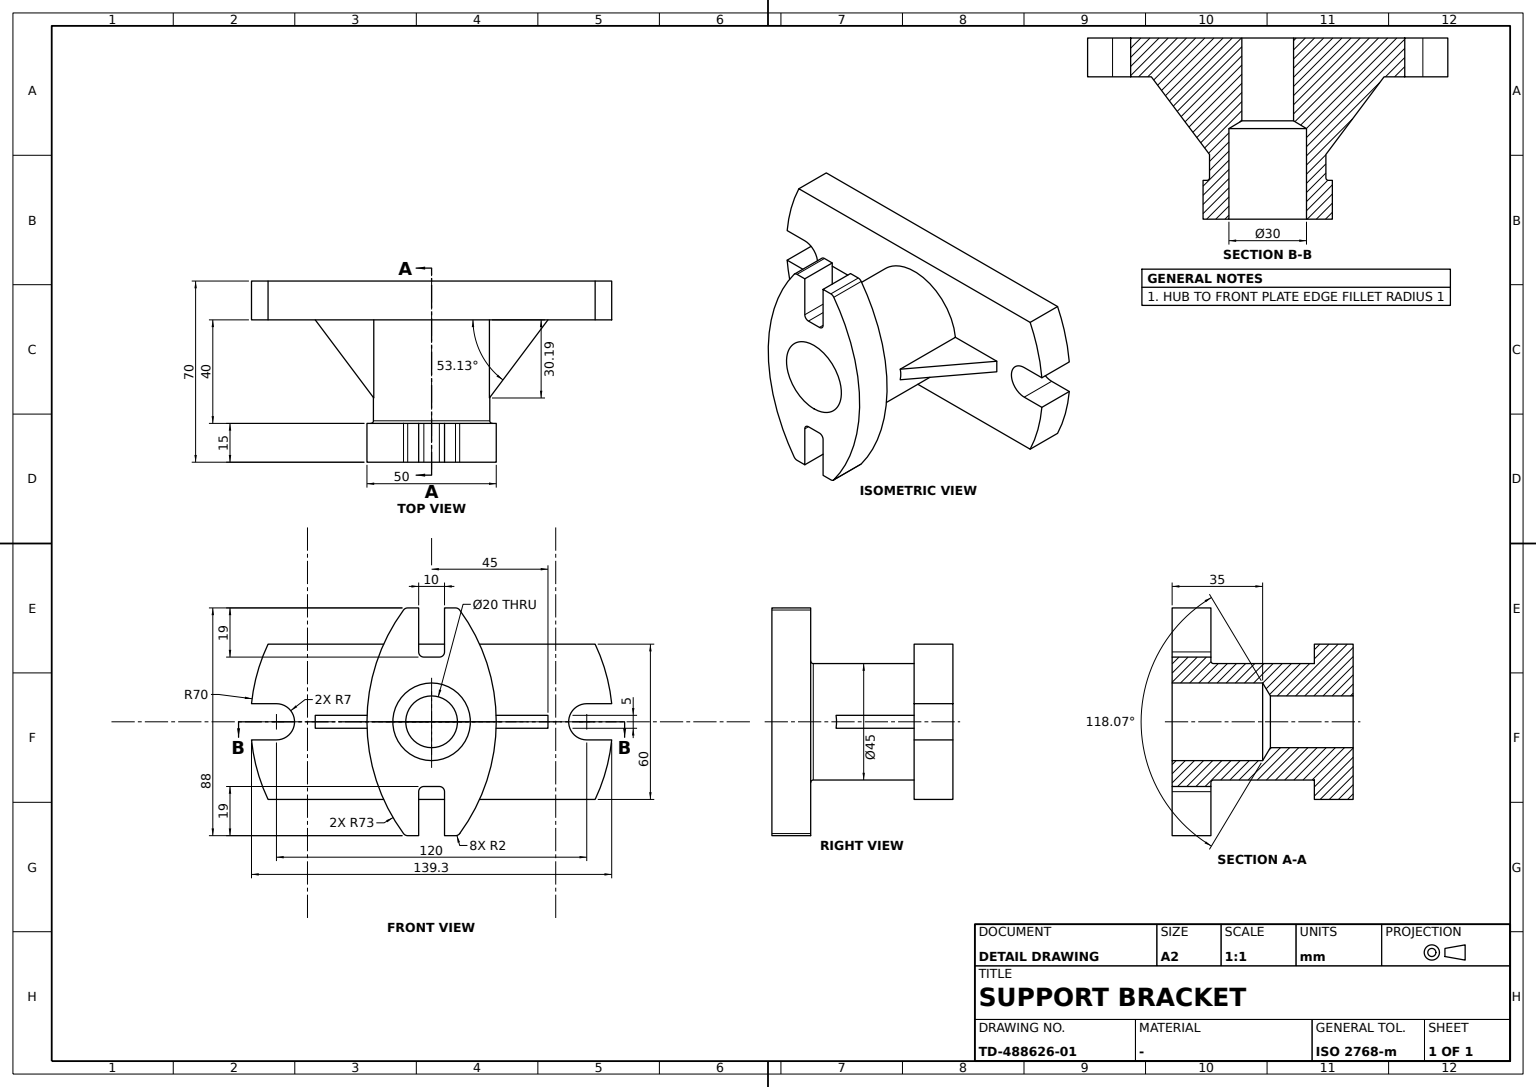
ISO-10303-21;
HEADER;
FILE_DESCRIPTION((''),'2;1');
FILE_NAME('','',(''),(''),'','','');
FILE_SCHEMA(('AUTOMOTIVE_DESIGN'));
ENDSEC;
DATA;
#1=APPLICATION_CONTEXT('');
#2=PRODUCT_CONTEXT('',#1,'mechanical');
#3=PRODUCT('','','',(#2));
#4=PRODUCT_DEFINITION_FORMATION('','',#3);
#5=PRODUCT_DEFINITION_CONTEXT('',#1,'design');
#6=PRODUCT_DEFINITION('','',#4,#5);
#7=PRODUCT_DEFINITION_SHAPE('','',#6);
#8=(LENGTH_UNIT()NAMED_UNIT(*)SI_UNIT(.MILLI.,.METRE.));
#9=(NAMED_UNIT(*)PLANE_ANGLE_UNIT()SI_UNIT($,.RADIAN.));
#10=(NAMED_UNIT(*)SI_UNIT($,.STERADIAN.)SOLID_ANGLE_UNIT());
#11=UNCERTAINTY_MEASURE_WITH_UNIT(LENGTH_MEASURE(0.005),#8,'distance_accuracy_value','');
#12=(GEOMETRIC_REPRESENTATION_CONTEXT(3)GLOBAL_UNCERTAINTY_ASSIGNED_CONTEXT((#11))GLOBAL_UNIT_ASSIGNED_CONTEXT((#8,#9,#10))REPRESENTATION_CONTEXT('',''));
#13=CARTESIAN_POINT('',(-7.5,-63.245553,30.));
#14=VERTEX_POINT('',#13);
#15=CARTESIAN_POINT('',(7.5,-63.245553,30.));
#16=VERTEX_POINT('',#15);
#17=DIRECTION('',(1.,0.,0.));
#18=VECTOR('',#17,1000.);
#19=LINE('',#13,#18);
#20=EDGE_CURVE('',#14,#16,#19,.T.);
#21=ORIENTED_EDGE('',*,*,#20,.F.);
#22=CARTESIAN_POINT('',(-7.5,-69.649121,7.));
#23=VERTEX_POINT('',#22);
#24=CARTESIAN_POINT('',(-7.5,0.,0.));
#25=DIRECTION('',(0.,0.,-1.));
#26=AXIS2_PLACEMENT_3D('',#24,#17,#25);
#27=CIRCLE('',#26,70.);
#28=EDGE_CURVE('',#14,#23,#27,.T.);
#29=ORIENTED_EDGE('',*,*,#28,.T.);
#30=CARTESIAN_POINT('',(7.5,-69.649121,7.));
#31=VERTEX_POINT('',#30);
#32=LINE('',#22,#18);
#33=EDGE_CURVE('',#23,#31,#32,.T.);
#34=ORIENTED_EDGE('',*,*,#33,.T.);
#35=CARTESIAN_POINT('',(7.5,0.,0.));
#36=AXIS2_PLACEMENT_3D('',#35,#17,#25);
#37=CIRCLE('',#36,70.);
#38=EDGE_CURVE('',#16,#31,#37,.T.);
#39=ORIENTED_EDGE('',*,*,#38,.F.);
#40=EDGE_LOOP('',(#21,#29,#34,#39));
#41=FACE_BOUND('',#40,.T.);
#42=CARTESIAN_POINT('',(0.,0.,0.));
#43=DIRECTION('',(0.,1.,0.));
#44=AXIS2_PLACEMENT_3D('',#42,#17,#43);
#45=CYLINDRICAL_SURFACE('',#44,70.);
#46=ADVANCED_FACE('',(#41),#45,.T.);
#47=CARTESIAN_POINT('',(7.5,63.245553,-30.));
#48=VERTEX_POINT('',#47);
#49=CARTESIAN_POINT('',(7.5,69.649121,-7.));
#50=VERTEX_POINT('',#49);
#51=EDGE_CURVE('',#48,#50,#37,.T.);
#52=ORIENTED_EDGE('',*,*,#51,.F.);
#53=CARTESIAN_POINT('',(-7.5,63.245553,-30.));
#54=VERTEX_POINT('',#53);
#55=LINE('',#53,#18);
#56=EDGE_CURVE('',#54,#48,#55,.T.);
#57=ORIENTED_EDGE('',*,*,#56,.F.);
#58=CARTESIAN_POINT('',(-7.5,69.649121,-7.));
#59=VERTEX_POINT('',#58);
#60=EDGE_CURVE('',#54,#59,#27,.T.);
#61=ORIENTED_EDGE('',*,*,#60,.T.);
#62=LINE('',#58,#18);
#63=EDGE_CURVE('',#59,#50,#62,.T.);
#64=ORIENTED_EDGE('',*,*,#63,.T.);
#65=EDGE_LOOP('',(#52,#57,#61,#64));
#66=FACE_BOUND('',#65,.T.);
#67=ADVANCED_FACE('',(#66),#45,.T.);
#68=CARTESIAN_POINT('',(62.5,-5.,-44.));
#69=VERTEX_POINT('',#68);
#70=CARTESIAN_POINT('',(47.5,-5.,-44.));
#71=VERTEX_POINT('',#70);
#72=DIRECTION('',(-1.,0.,0.));
#73=VECTOR('',#72,1000.);
#74=LINE('',#68,#73);
#75=EDGE_CURVE('',#69,#71,#74,.T.);
#76=ORIENTED_EDGE('',*,*,#75,.F.);
#77=CARTESIAN_POINT('',(62.5,-9.245087,-44.));
#78=VERTEX_POINT('',#77);
#79=CARTESIAN_POINT('',(62.5,0.,-44.));
#80=DIRECTION('',(0.,-1.,0.));
#81=VECTOR('',#80,1000.);
#82=LINE('',#79,#81);
#83=EDGE_CURVE('',#69,#78,#82,.T.);
#84=ORIENTED_EDGE('',*,*,#83,.T.);
#85=CARTESIAN_POINT('',(47.5,-9.245087,-44.));
#86=VERTEX_POINT('',#85);
#87=CARTESIAN_POINT('',(55.,-9.245087,-44.));
#88=LINE('',#87,#73);
#89=EDGE_CURVE('',#78,#86,#88,.T.);
#90=ORIENTED_EDGE('',*,*,#89,.T.);
#91=CARTESIAN_POINT('',(47.5,0.,-44.));
#92=LINE('',#91,#81);
#93=EDGE_CURVE('',#71,#86,#92,.T.);
#94=ORIENTED_EDGE('',*,*,#93,.F.);
#95=EDGE_LOOP('',(#76,#84,#90,#94));
#96=FACE_BOUND('',#95,.T.);
#97=CARTESIAN_POINT('',(62.5,5.,-44.));
#98=DIRECTION('',(0.,0.,1.));
#99=AXIS2_PLACEMENT_3D('',#97,#98,#43);
#100=PLANE('',#99);
#101=ADVANCED_FACE('',(#96),#100,.F.);
#102=VERTEX_POINT('',#97);
#103=CARTESIAN_POINT('',(47.5,5.,-44.));
#104=VERTEX_POINT('',#103);
#105=LINE('',#97,#73);
#106=EDGE_CURVE('',#102,#104,#105,.T.);
#107=ORIENTED_EDGE('',*,*,#106,.F.);
#108=CARTESIAN_POINT('',(62.5,5.,-27.));
#109=VERTEX_POINT('',#108);
#110=CARTESIAN_POINT('',(62.5,5.,-25.));
#111=VECTOR('',#25,1000.);
#112=LINE('',#110,#111);
#113=EDGE_CURVE('',#109,#102,#112,.T.);
#114=ORIENTED_EDGE('',*,*,#113,.F.);
#115=CARTESIAN_POINT('',(47.5,5.,-27.));
#116=VERTEX_POINT('',#115);
#117=CARTESIAN_POINT('',(55.,5.,-27.));
#118=LINE('',#117,#73);
#119=EDGE_CURVE('',#109,#116,#118,.T.);
#120=ORIENTED_EDGE('',*,*,#119,.T.);
#121=CARTESIAN_POINT('',(47.5,5.,-25.));
#122=LINE('',#121,#111);
#123=EDGE_CURVE('',#116,#104,#122,.T.);
#124=ORIENTED_EDGE('',*,*,#123,.T.);
#125=EDGE_LOOP('',(#107,#114,#120,#124));
#126=FACE_BOUND('',#125,.T.);
#127=AXIS2_PLACEMENT_3D('',#110,#43,#25);
#128=PLANE('',#127);
#129=ADVANCED_FACE('',(#126),#128,.F.);
#130=CARTESIAN_POINT('',(-7.5,0.,-10.));
#131=VERTEX_POINT('',#130);
#132=CIRCLE('',#26,10.);
#133=EDGE_CURVE('',#131,#131,#132,.T.);
#134=ORIENTED_EDGE('',*,*,#133,.F.);
#135=EDGE_LOOP('',(#134));
#136=FACE_BOUND('',#135,.T.);
#137=CARTESIAN_POINT('',(24.5,0.,-10.));
#138=VERTEX_POINT('',#137);
#139=CARTESIAN_POINT('',(24.5,0.,0.));
#140=AXIS2_PLACEMENT_3D('',#139,#17,#25);
#141=CIRCLE('',#140,10.);
#142=EDGE_CURVE('',#138,#138,#141,.T.);
#143=ORIENTED_EDGE('',*,*,#142,.T.);
#144=EDGE_LOOP('',(#143));
#145=FACE_BOUND('',#144,.T.);
#146=CARTESIAN_POINT('',(27.5,0.,0.));
#147=AXIS2_PLACEMENT_3D('',#146,#17,#43);
#148=CYLINDRICAL_SURFACE('',#147,10.);
#149=ADVANCED_FACE('',(#136,#145),#148,.F.);
#150=CARTESIAN_POINT('',(62.5,-3.,25.));
#151=VERTEX_POINT('',#150);
#152=CARTESIAN_POINT('',(62.5,3.,25.));
#153=VERTEX_POINT('',#152);
#154=CARTESIAN_POINT('',(62.5,-5.,25.));
#155=VECTOR('',#43,1000.);
#156=LINE('',#154,#155);
#157=EDGE_CURVE('',#151,#153,#156,.T.);
#158=ORIENTED_EDGE('',*,*,#157,.T.);
#159=CARTESIAN_POINT('',(47.5,3.,25.));
#160=VERTEX_POINT('',#159);
#161=CARTESIAN_POINT('',(55.,3.,25.));
#162=LINE('',#161,#73);
#163=EDGE_CURVE('',#153,#160,#162,.T.);
#164=ORIENTED_EDGE('',*,*,#163,.T.);
#165=CARTESIAN_POINT('',(47.5,-3.,25.));
#166=VERTEX_POINT('',#165);
#167=CARTESIAN_POINT('',(47.5,-5.,25.));
#168=LINE('',#167,#155);
#169=EDGE_CURVE('',#166,#160,#168,.T.);
#170=ORIENTED_EDGE('',*,*,#169,.F.);
#171=CARTESIAN_POINT('',(55.,-3.,25.));
#172=LINE('',#171,#73);
#173=EDGE_CURVE('',#151,#166,#172,.T.);
#174=ORIENTED_EDGE('',*,*,#173,.F.);
#175=EDGE_LOOP('',(#158,#164,#170,#174));
#176=FACE_BOUND('',#175,.T.);
#177=AXIS2_PLACEMENT_3D('',#154,#98,#43);
#178=PLANE('',#177);
#179=ADVANCED_FACE('',(#176),#178,.T.);
#180=ORIENTED_EDGE('',*,*,#173,.T.);
#181=CARTESIAN_POINT('',(47.5,-5.,27.));
#182=VERTEX_POINT('',#181);
#183=CARTESIAN_POINT('',(47.5,-3.,27.));
#184=AXIS2_PLACEMENT_3D('',#183,#17,#25);
#185=CIRCLE('',#184,2.);
#186=EDGE_CURVE('',#182,#166,#185,.T.);
#187=ORIENTED_EDGE('',*,*,#186,.F.);
#188=CARTESIAN_POINT('',(62.5,-5.,27.));
#189=VERTEX_POINT('',#188);
#190=CARTESIAN_POINT('',(55.,-5.,27.));
#191=LINE('',#190,#73);
#192=EDGE_CURVE('',#189,#182,#191,.T.);
#193=ORIENTED_EDGE('',*,*,#192,.F.);
#194=CARTESIAN_POINT('',(62.5,-3.,27.));
#195=AXIS2_PLACEMENT_3D('',#194,#17,#25);
#196=CIRCLE('',#195,2.);
#197=EDGE_CURVE('',#189,#151,#196,.T.);
#198=ORIENTED_EDGE('',*,*,#197,.T.);
#199=EDGE_LOOP('',(#180,#187,#193,#198));
#200=FACE_BOUND('',#199,.T.);
#201=CARTESIAN_POINT('',(55.,-3.,27.));
#202=AXIS2_PLACEMENT_3D('',#201,#72,#25);
#203=CYLINDRICAL_SURFACE('',#202,2.);
#204=ADVANCED_FACE('',(#200),#203,.F.);
#205=CARTESIAN_POINT('',(47.5,-5.,-27.));
#206=VERTEX_POINT('',#205);
#207=CARTESIAN_POINT('',(47.5,-5.,0.));
#208=LINE('',#207,#111);
#209=EDGE_CURVE('',#206,#71,#208,.T.);
#210=ORIENTED_EDGE('',*,*,#209,.F.);
#211=CARTESIAN_POINT('',(62.5,-5.,-27.));
#212=VERTEX_POINT('',#211);
#213=CARTESIAN_POINT('',(55.,-5.,-27.));
#214=LINE('',#213,#73);
#215=EDGE_CURVE('',#212,#206,#214,.T.);
#216=ORIENTED_EDGE('',*,*,#215,.F.);
#217=CARTESIAN_POINT('',(62.5,-5.,0.));
#218=LINE('',#217,#111);
#219=EDGE_CURVE('',#212,#69,#218,.T.);
#220=ORIENTED_EDGE('',*,*,#219,.T.);
#221=ORIENTED_EDGE('',*,*,#75,.T.);
#222=EDGE_LOOP('',(#210,#216,#220,#221));
#223=FACE_BOUND('',#222,.T.);
#224=AXIS2_PLACEMENT_3D('',#154,#80,#98);
#225=PLANE('',#224);
#226=ADVANCED_FACE('',(#223),#225,.F.);
#227=CARTESIAN_POINT('',(62.5,5.,27.));
#228=VERTEX_POINT('',#227);
#229=CARTESIAN_POINT('',(47.5,5.,27.));
#230=VERTEX_POINT('',#229);
#231=CARTESIAN_POINT('',(55.,5.,27.));
#232=LINE('',#231,#73);
#233=EDGE_CURVE('',#228,#230,#232,.T.);
#234=ORIENTED_EDGE('',*,*,#233,.T.);
#235=CARTESIAN_POINT('',(47.5,3.,27.));
#236=AXIS2_PLACEMENT_3D('',#235,#17,#25);
#237=CIRCLE('',#236,2.);
#238=EDGE_CURVE('',#160,#230,#237,.T.);
#239=ORIENTED_EDGE('',*,*,#238,.F.);
#240=ORIENTED_EDGE('',*,*,#163,.F.);
#241=CARTESIAN_POINT('',(62.5,3.,27.));
#242=AXIS2_PLACEMENT_3D('',#241,#17,#25);
#243=CIRCLE('',#242,2.);
#244=EDGE_CURVE('',#153,#228,#243,.T.);
#245=ORIENTED_EDGE('',*,*,#244,.T.);
#246=EDGE_LOOP('',(#234,#239,#240,#245));
#247=FACE_BOUND('',#246,.T.);
#248=CARTESIAN_POINT('',(55.,3.,27.));
#249=AXIS2_PLACEMENT_3D('',#248,#72,#43);
#250=CYLINDRICAL_SURFACE('',#249,2.);
#251=ADVANCED_FACE('',(#247),#250,.F.);
#252=CARTESIAN_POINT('',(7.5,22.36068,-2.5));
#253=VERTEX_POINT('',#252);
#254=CARTESIAN_POINT('',(7.5,45.,-2.5));
#255=VERTEX_POINT('',#254);
#256=CARTESIAN_POINT('',(7.5,0.,-2.5));
#257=LINE('',#256,#155);
#258=EDGE_CURVE('',#253,#255,#257,.T.);
#259=ORIENTED_EDGE('',*,*,#258,.T.);
#260=CARTESIAN_POINT('',(37.68576,22.36068,-2.5));
#261=VERTEX_POINT('',#260);
#262=DIRECTION('',(0.8,-0.6,0.));
#263=VECTOR('',#262,1000.);
#264=LINE('',#254,#263);
#265=EDGE_CURVE('',#255,#261,#264,.T.);
#266=ORIENTED_EDGE('',*,*,#265,.T.);
#267=LINE('',#252,#18);
#268=EDGE_CURVE('',#253,#261,#267,.T.);
#269=ORIENTED_EDGE('',*,*,#268,.F.);
#270=EDGE_LOOP('',(#259,#266,#269));
#271=FACE_BOUND('',#270,.T.);
#272=CARTESIAN_POINT('',(0.,0.,-2.5));
#273=AXIS2_PLACEMENT_3D('',#272,#98,#17);
#274=PLANE('',#273);
#275=ADVANCED_FACE('',(#271),#274,.F.);
#276=CARTESIAN_POINT('',(62.5,-10.857625,-43.183099));
#277=VERTEX_POINT('',#276);
#278=CARTESIAN_POINT('',(47.5,-10.857625,-43.183099));
#279=VERTEX_POINT('',#278);
#280=CARTESIAN_POINT('',(55.,-10.857625,-43.183099));
#281=LINE('',#280,#18);
#282=EDGE_CURVE('',#277,#279,#281,.F.);
#283=ORIENTED_EDGE('',*,*,#282,.F.);
#284=CARTESIAN_POINT('',(62.5,-10.857625,43.183099));
#285=VERTEX_POINT('',#284);
#286=CARTESIAN_POINT('',(62.5,48.,0.));
#287=AXIS2_PLACEMENT_3D('',#286,#17,#25);
#288=CIRCLE('',#287,73.);
#289=EDGE_CURVE('',#285,#277,#288,.T.);
#290=ORIENTED_EDGE('',*,*,#289,.F.);
#291=CARTESIAN_POINT('',(47.5,-10.857625,43.183099));
#292=VERTEX_POINT('',#291);
#293=CARTESIAN_POINT('',(55.,-10.857625,43.183099));
#294=LINE('',#293,#18);
#295=EDGE_CURVE('',#292,#285,#294,.T.);
#296=ORIENTED_EDGE('',*,*,#295,.F.);
#297=CARTESIAN_POINT('',(47.5,48.,0.));
#298=AXIS2_PLACEMENT_3D('',#297,#17,#25);
#299=CIRCLE('',#298,73.);
#300=EDGE_CURVE('',#292,#279,#299,.T.);
#301=ORIENTED_EDGE('',*,*,#300,.T.);
#302=EDGE_LOOP('',(#283,#290,#296,#301));
#303=FACE_BOUND('',#302,.T.);
#304=CARTESIAN_POINT('',(55.,48.,0.));
#305=AXIS2_PLACEMENT_3D('',#304,#17,#43);
#306=CYLINDRICAL_SURFACE('',#305,73.);
#307=ADVANCED_FACE('',(#303),#306,.T.);
#308=CARTESIAN_POINT('',(47.5,-5.,44.));
#309=VERTEX_POINT('',#308);
#310=CARTESIAN_POINT('',(47.5,-9.245087,44.));
#311=VERTEX_POINT('',#310);
#312=CARTESIAN_POINT('',(47.5,0.,44.));
#313=LINE('',#312,#81);
#314=EDGE_CURVE('',#309,#311,#313,.T.);
#315=ORIENTED_EDGE('',*,*,#314,.T.);
#316=CARTESIAN_POINT('',(62.5,-9.245087,44.));
#317=VERTEX_POINT('',#316);
#318=CARTESIAN_POINT('',(55.,-9.245087,44.));
#319=LINE('',#318,#18);
#320=EDGE_CURVE('',#311,#317,#319,.T.);
#321=ORIENTED_EDGE('',*,*,#320,.T.);
#322=CARTESIAN_POINT('',(62.5,-5.,44.));
#323=VERTEX_POINT('',#322);
#324=CARTESIAN_POINT('',(62.5,0.,44.));
#325=LINE('',#324,#81);
#326=EDGE_CURVE('',#323,#317,#325,.T.);
#327=ORIENTED_EDGE('',*,*,#326,.F.);
#328=LINE('',#322,#73);
#329=EDGE_CURVE('',#323,#309,#328,.T.);
#330=ORIENTED_EDGE('',*,*,#329,.T.);
#331=EDGE_LOOP('',(#315,#321,#327,#330));
#332=FACE_BOUND('',#331,.T.);
#333=CARTESIAN_POINT('',(62.5,5.,44.));
#334=AXIS2_PLACEMENT_3D('',#333,#98,#43);
#335=PLANE('',#334);
#336=ADVANCED_FACE('',(#332),#335,.T.);
#337=CARTESIAN_POINT('',(7.5,-45.,2.5));
#338=VERTEX_POINT('',#337);
#339=CARTESIAN_POINT('',(7.5,-22.36068,2.5));
#340=VERTEX_POINT('',#339);
#341=CARTESIAN_POINT('',(7.5,0.,2.5));
#342=LINE('',#341,#155);
#343=EDGE_CURVE('',#338,#340,#342,.T.);
#344=ORIENTED_EDGE('',*,*,#343,.T.);
#345=CARTESIAN_POINT('',(7.5,22.36068,2.5));
#346=VERTEX_POINT('',#345);
#347=CIRCLE('',#36,22.5);
#348=EDGE_CURVE('',#346,#340,#347,.T.);
#349=ORIENTED_EDGE('',*,*,#348,.F.);
#350=CARTESIAN_POINT('',(7.5,45.,2.5));
#351=VERTEX_POINT('',#350);
#352=EDGE_CURVE('',#346,#351,#342,.T.);
#353=ORIENTED_EDGE('',*,*,#352,.T.);
#354=CARTESIAN_POINT('',(7.5,45.,0.));
#355=LINE('',#354,#111);
#356=EDGE_CURVE('',#351,#255,#355,.T.);
#357=ORIENTED_EDGE('',*,*,#356,.T.);
#358=ORIENTED_EDGE('',*,*,#258,.F.);
#359=CARTESIAN_POINT('',(7.5,-22.36068,-2.5));
#360=VERTEX_POINT('',#359);
#361=EDGE_CURVE('',#360,#253,#347,.T.);
#362=ORIENTED_EDGE('',*,*,#361,.F.);
#363=CARTESIAN_POINT('',(7.5,-45.,-2.5));
#364=VERTEX_POINT('',#363);
#365=EDGE_CURVE('',#364,#360,#257,.T.);
#366=ORIENTED_EDGE('',*,*,#365,.F.);
#367=CARTESIAN_POINT('',(7.5,-45.,0.));
#368=VECTOR('',#98,1000.);
#369=LINE('',#367,#368);
#370=EDGE_CURVE('',#364,#338,#369,.T.);
#371=ORIENTED_EDGE('',*,*,#370,.T.);
#372=EDGE_LOOP('',(#344,#349,#353,#357,#358,#362,#366,#371));
#373=FACE_BOUND('',#372,.T.);
#374=CARTESIAN_POINT('',(7.5,-63.245553,-30.));
#375=VERTEX_POINT('',#374);
#376=CARTESIAN_POINT('',(7.5,0.,-30.));
#377=LINE('',#376,#81);
#378=EDGE_CURVE('',#48,#375,#377,.T.);
#379=ORIENTED_EDGE('',*,*,#378,.F.);
#380=ORIENTED_EDGE('',*,*,#51,.T.);
#381=CARTESIAN_POINT('',(7.5,60.,-7.));
#382=VERTEX_POINT('',#381);
#383=CARTESIAN_POINT('',(7.5,-60.,-7.));
#384=LINE('',#383,#155);
#385=EDGE_CURVE('',#382,#50,#384,.T.);
#386=ORIENTED_EDGE('',*,*,#385,.F.);
#387=CARTESIAN_POINT('',(7.5,60.,7.));
#388=VERTEX_POINT('',#387);
#389=CARTESIAN_POINT('',(7.5,60.,0.));
#390=AXIS2_PLACEMENT_3D('',#389,#17,#25);
#391=CIRCLE('',#390,7.);
#392=EDGE_CURVE('',#388,#382,#391,.T.);
#393=ORIENTED_EDGE('',*,*,#392,.F.);
#394=CARTESIAN_POINT('',(7.5,69.649121,7.));
#395=VERTEX_POINT('',#394);
#396=CARTESIAN_POINT('',(7.5,0.,7.));
#397=LINE('',#396,#155);
#398=EDGE_CURVE('',#388,#395,#397,.T.);
#399=ORIENTED_EDGE('',*,*,#398,.T.);
#400=CARTESIAN_POINT('',(7.5,63.245553,30.));
#401=VERTEX_POINT('',#400);
#402=EDGE_CURVE('',#395,#401,#37,.T.);
#403=ORIENTED_EDGE('',*,*,#402,.T.);
#404=CARTESIAN_POINT('',(7.5,0.,30.));
#405=LINE('',#404,#155);
#406=EDGE_CURVE('',#16,#401,#405,.T.);
#407=ORIENTED_EDGE('',*,*,#406,.F.);
#408=ORIENTED_EDGE('',*,*,#38,.T.);
#409=CARTESIAN_POINT('',(7.5,-60.,7.));
#410=VERTEX_POINT('',#409);
#411=LINE('',#387,#81);
#412=EDGE_CURVE('',#410,#31,#411,.T.);
#413=ORIENTED_EDGE('',*,*,#412,.F.);
#414=VERTEX_POINT('',#383);
#415=CARTESIAN_POINT('',(7.5,-60.,0.));
#416=AXIS2_PLACEMENT_3D('',#415,#17,#25);
#417=CIRCLE('',#416,7.);
#418=EDGE_CURVE('',#414,#410,#417,.T.);
#419=ORIENTED_EDGE('',*,*,#418,.F.);
#420=CARTESIAN_POINT('',(7.5,-69.649121,-7.));
#421=VERTEX_POINT('',#420);
#422=CARTESIAN_POINT('',(7.5,0.,-7.));
#423=LINE('',#422,#81);
#424=EDGE_CURVE('',#414,#421,#423,.T.);
#425=ORIENTED_EDGE('',*,*,#424,.T.);
#426=EDGE_CURVE('',#421,#375,#37,.T.);
#427=ORIENTED_EDGE('',*,*,#426,.T.);
#428=EDGE_LOOP('',(#379,#380,#386,#393,#399,#403,#407,#408,#413,#419,#425,#427));
#429=FACE_BOUND('',#428,.T.);
#430=AXIS2_PLACEMENT_3D('',#35,#17,#43);
#431=PLANE('',#430);
#432=ADVANCED_FACE('',(#373,#429),#431,.T.);
#433=ORIENTED_EDGE('',*,*,#385,.T.);
#434=ORIENTED_EDGE('',*,*,#63,.F.);
#435=CARTESIAN_POINT('',(-7.5,60.,-7.));
#436=VERTEX_POINT('',#435);
#437=CARTESIAN_POINT('',(-7.5,-60.,-7.));
#438=LINE('',#437,#155);
#439=EDGE_CURVE('',#436,#59,#438,.T.);
#440=ORIENTED_EDGE('',*,*,#439,.F.);
#441=CARTESIAN_POINT('',(0.,60.,-7.));
#442=LINE('',#441,#18);
#443=EDGE_CURVE('',#436,#382,#442,.T.);
#444=ORIENTED_EDGE('',*,*,#443,.T.);
#445=EDGE_LOOP('',(#433,#434,#440,#444));
#446=FACE_BOUND('',#445,.T.);
#447=CARTESIAN_POINT('',(0.,-60.,-7.));
#448=AXIS2_PLACEMENT_3D('',#447,#98,#80);
#449=PLANE('',#448);
#450=ADVANCED_FACE('',(#446),#449,.T.);
#451=CARTESIAN_POINT('',(62.5,0.,-15.));
#452=VERTEX_POINT('',#451);
#453=CARTESIAN_POINT('',(62.5,0.,0.));
#454=AXIS2_PLACEMENT_3D('',#453,#17,#25);
#455=CIRCLE('',#454,15.);
#456=EDGE_CURVE('',#452,#452,#455,.T.);
#457=ORIENTED_EDGE('',*,*,#456,.T.);
#458=EDGE_LOOP('',(#457));
#459=FACE_BOUND('',#458,.T.);
#460=CARTESIAN_POINT('',(27.5,0.,-15.));
#461=VERTEX_POINT('',#460);
#462=AXIS2_PLACEMENT_3D('',#146,#17,#25);
#463=CIRCLE('',#462,15.);
#464=EDGE_CURVE('',#461,#461,#463,.T.);
#465=ORIENTED_EDGE('',*,*,#464,.F.);
#466=EDGE_LOOP('',(#465));
#467=FACE_BOUND('',#466,.T.);
#468=CARTESIAN_POINT('',(55.,0.,0.));
#469=AXIS2_PLACEMENT_3D('',#468,#17,#43);
#470=CYLINDRICAL_SURFACE('',#469,15.);
#471=ADVANCED_FACE('',(#459,#467),#470,.F.);
#472=CARTESIAN_POINT('',(62.5,-3.,-25.));
#473=VERTEX_POINT('',#472);
#474=CARTESIAN_POINT('',(62.5,-3.,-27.));
#475=AXIS2_PLACEMENT_3D('',#474,#17,#25);
#476=CIRCLE('',#475,2.);
#477=EDGE_CURVE('',#473,#212,#476,.T.);
#478=ORIENTED_EDGE('',*,*,#477,.T.);
#479=ORIENTED_EDGE('',*,*,#215,.T.);
#480=CARTESIAN_POINT('',(47.5,-3.,-25.));
#481=VERTEX_POINT('',#480);
#482=CARTESIAN_POINT('',(47.5,-3.,-27.));
#483=AXIS2_PLACEMENT_3D('',#482,#17,#25);
#484=CIRCLE('',#483,2.);
#485=EDGE_CURVE('',#481,#206,#484,.T.);
#486=ORIENTED_EDGE('',*,*,#485,.F.);
#487=CARTESIAN_POINT('',(55.,-3.,-25.));
#488=LINE('',#487,#73);
#489=EDGE_CURVE('',#473,#481,#488,.T.);
#490=ORIENTED_EDGE('',*,*,#489,.F.);
#491=EDGE_LOOP('',(#478,#479,#486,#490));
#492=FACE_BOUND('',#491,.T.);
#493=CARTESIAN_POINT('',(55.,-3.,-27.));
#494=AXIS2_PLACEMENT_3D('',#493,#72,#80);
#495=CYLINDRICAL_SURFACE('',#494,2.);
#496=ADVANCED_FACE('',(#492),#495,.F.);
#497=ORIENTED_EDGE('',*,*,#56,.T.);
#498=ORIENTED_EDGE('',*,*,#378,.T.);
#499=CARTESIAN_POINT('',(-7.5,-63.245553,-30.));
#500=VERTEX_POINT('',#499);
#501=LINE('',#499,#18);
#502=EDGE_CURVE('',#500,#375,#501,.T.);
#503=ORIENTED_EDGE('',*,*,#502,.F.);
#504=CARTESIAN_POINT('',(-7.5,0.,-30.));
#505=LINE('',#504,#81);
#506=EDGE_CURVE('',#54,#500,#505,.T.);
#507=ORIENTED_EDGE('',*,*,#506,.F.);
#508=EDGE_LOOP('',(#497,#498,#503,#507));
#509=FACE_BOUND('',#508,.T.);
#510=CARTESIAN_POINT('',(0.,63.245553,-30.));
#511=AXIS2_PLACEMENT_3D('',#510,#98,#80);
#512=PLANE('',#511);
#513=ADVANCED_FACE('',(#509),#512,.F.);
#514=ORIENTED_EDGE('',*,*,#443,.F.);
#515=CARTESIAN_POINT('',(-7.5,60.,7.));
#516=VERTEX_POINT('',#515);
#517=CARTESIAN_POINT('',(-7.5,60.,0.));
#518=AXIS2_PLACEMENT_3D('',#517,#17,#25);
#519=CIRCLE('',#518,7.);
#520=EDGE_CURVE('',#516,#436,#519,.T.);
#521=ORIENTED_EDGE('',*,*,#520,.F.);
#522=CARTESIAN_POINT('',(0.,60.,7.));
#523=LINE('',#522,#18);
#524=EDGE_CURVE('',#516,#388,#523,.T.);
#525=ORIENTED_EDGE('',*,*,#524,.T.);
#526=ORIENTED_EDGE('',*,*,#392,.T.);
#527=EDGE_LOOP('',(#514,#521,#525,#526));
#528=FACE_BOUND('',#527,.T.);
#529=CARTESIAN_POINT('',(0.,60.,0.));
#530=AXIS2_PLACEMENT_3D('',#529,#17,#43);
#531=CYLINDRICAL_SURFACE('',#530,7.);
#532=ADVANCED_FACE('',(#528),#531,.F.);
#533=ORIENTED_EDGE('',*,*,#106,.T.);
#534=CARTESIAN_POINT('',(47.5,9.245087,-44.));
#535=VERTEX_POINT('',#534);
#536=LINE('',#103,#155);
#537=EDGE_CURVE('',#104,#535,#536,.T.);
#538=ORIENTED_EDGE('',*,*,#537,.T.);
#539=CARTESIAN_POINT('',(62.5,9.245087,-44.));
#540=VERTEX_POINT('',#539);
#541=CARTESIAN_POINT('',(55.,9.245087,-44.));
#542=LINE('',#541,#73);
#543=EDGE_CURVE('',#540,#535,#542,.T.);
#544=ORIENTED_EDGE('',*,*,#543,.F.);
#545=LINE('',#97,#155);
#546=EDGE_CURVE('',#102,#540,#545,.T.);
#547=ORIENTED_EDGE('',*,*,#546,.F.);
#548=EDGE_LOOP('',(#533,#538,#544,#547));
#549=FACE_BOUND('',#548,.T.);
#550=ADVANCED_FACE('',(#549),#100,.F.);
#551=ORIENTED_EDGE('',*,*,#361,.T.);
#552=ORIENTED_EDGE('',*,*,#268,.T.);
#553=CARTESIAN_POINT('',(37.68576,22.36068,2.5));
#554=VERTEX_POINT('',#553);
#555=CARTESIAN_POINT('',(67.5,0.,0.));
#556=DIRECTION('',(0.6,0.8,0.));
#557=AXIS2_PLACEMENT_3D('',#555,#556,#262);
#558=ELLIPSE('',#557,37.5,22.5);
#559=EDGE_CURVE('',#261,#554,#558,.T.);
#560=ORIENTED_EDGE('',*,*,#559,.T.);
#561=LINE('',#345,#18);
#562=EDGE_CURVE('',#346,#554,#561,.T.);
#563=ORIENTED_EDGE('',*,*,#562,.F.);
#564=ORIENTED_EDGE('',*,*,#348,.T.);
#565=CARTESIAN_POINT('',(37.68576,-22.36068,2.5));
#566=VERTEX_POINT('',#565);
#567=LINE('',#339,#18);
#568=EDGE_CURVE('',#340,#566,#567,.T.);
#569=ORIENTED_EDGE('',*,*,#568,.T.);
#570=CARTESIAN_POINT('',(37.68576,-22.36068,-2.5));
#571=VERTEX_POINT('',#570);
#572=DIRECTION('',(0.6,-0.8,0.));
#573=DIRECTION('',(0.8,0.6,0.));
#574=AXIS2_PLACEMENT_3D('',#555,#572,#573);
#575=ELLIPSE('',#574,37.5,22.5);
#576=EDGE_CURVE('',#566,#571,#575,.T.);
#577=ORIENTED_EDGE('',*,*,#576,.T.);
#578=LINE('',#359,#18);
#579=EDGE_CURVE('',#360,#571,#578,.T.);
#580=ORIENTED_EDGE('',*,*,#579,.F.);
#581=EDGE_LOOP('',(#551,#552,#560,#563,#564,#569,#577,#580));
#582=FACE_BOUND('',#581,.T.);
#583=CARTESIAN_POINT('',(46.5,0.,-22.5));
#584=VERTEX_POINT('',#583);
#585=CARTESIAN_POINT('',(46.5,0.,0.));
#586=AXIS2_PLACEMENT_3D('',#585,#17,#25);
#587=CIRCLE('',#586,22.5);
#588=EDGE_CURVE('',#584,#584,#587,.T.);
#589=ORIENTED_EDGE('',*,*,#588,.F.);
#590=EDGE_LOOP('',(#589));
#591=FACE_BOUND('',#590,.T.);
#592=CYLINDRICAL_SURFACE('',#147,22.5);
#593=ADVANCED_FACE('',(#582,#591),#592,.T.);
#594=CARTESIAN_POINT('',(62.5,3.,-25.));
#595=VERTEX_POINT('',#594);
#596=CARTESIAN_POINT('',(47.5,3.,-25.));
#597=VERTEX_POINT('',#596);
#598=CARTESIAN_POINT('',(55.,3.,-25.));
#599=LINE('',#598,#73);
#600=EDGE_CURVE('',#595,#597,#599,.T.);
#601=ORIENTED_EDGE('',*,*,#600,.T.);
#602=CARTESIAN_POINT('',(47.5,3.,-27.));
#603=AXIS2_PLACEMENT_3D('',#602,#17,#25);
#604=CIRCLE('',#603,2.);
#605=EDGE_CURVE('',#116,#597,#604,.T.);
#606=ORIENTED_EDGE('',*,*,#605,.F.);
#607=ORIENTED_EDGE('',*,*,#119,.F.);
#608=CARTESIAN_POINT('',(62.5,3.,-27.));
#609=AXIS2_PLACEMENT_3D('',#608,#17,#25);
#610=CIRCLE('',#609,2.);
#611=EDGE_CURVE('',#109,#595,#610,.T.);
#612=ORIENTED_EDGE('',*,*,#611,.T.);
#613=EDGE_LOOP('',(#601,#606,#607,#612));
#614=FACE_BOUND('',#613,.T.);
#615=CARTESIAN_POINT('',(55.,3.,-27.));
#616=AXIS2_PLACEMENT_3D('',#615,#72,#98);
#617=CYLINDRICAL_SURFACE('',#616,2.);
#618=ADVANCED_FACE('',(#614),#617,.F.);
#619=CARTESIAN_POINT('',(47.5,5.,44.));
#620=VERTEX_POINT('',#619);
#621=CARTESIAN_POINT('',(47.5,5.,0.));
#622=LINE('',#621,#368);
#623=EDGE_CURVE('',#230,#620,#622,.T.);
#624=ORIENTED_EDGE('',*,*,#623,.F.);
#625=ORIENTED_EDGE('',*,*,#233,.F.);
#626=VERTEX_POINT('',#333);
#627=CARTESIAN_POINT('',(62.5,5.,0.));
#628=LINE('',#627,#368);
#629=EDGE_CURVE('',#228,#626,#628,.T.);
#630=ORIENTED_EDGE('',*,*,#629,.T.);
#631=LINE('',#333,#73);
#632=EDGE_CURVE('',#626,#620,#631,.T.);
#633=ORIENTED_EDGE('',*,*,#632,.T.);
#634=EDGE_LOOP('',(#624,#625,#630,#633));
#635=FACE_BOUND('',#634,.T.);
#636=ADVANCED_FACE('',(#635),#128,.F.);
#637=ORIENTED_EDGE('',*,*,#559,.F.);
#638=ORIENTED_EDGE('',*,*,#265,.F.);
#639=ORIENTED_EDGE('',*,*,#356,.F.);
#640=LINE('',#350,#263);
#641=EDGE_CURVE('',#351,#554,#640,.T.);
#642=ORIENTED_EDGE('',*,*,#641,.T.);
#643=EDGE_LOOP('',(#637,#638,#639,#642));
#644=FACE_BOUND('',#643,.T.);
#645=DIRECTION('',(-0.8,0.6,0.));
#646=AXIS2_PLACEMENT_3D('',#354,#556,#645);
#647=PLANE('',#646);
#648=ADVANCED_FACE('',(#644),#647,.T.);
#649=VERTEX_POINT('',#437);
#650=CARTESIAN_POINT('',(-7.5,-69.649121,-7.));
#651=VERTEX_POINT('',#650);
#652=CARTESIAN_POINT('',(-7.5,0.,-7.));
#653=LINE('',#652,#81);
#654=EDGE_CURVE('',#649,#651,#653,.T.);
#655=ORIENTED_EDGE('',*,*,#654,.T.);
#656=LINE('',#650,#18);
#657=EDGE_CURVE('',#651,#421,#656,.T.);
#658=ORIENTED_EDGE('',*,*,#657,.T.);
#659=ORIENTED_EDGE('',*,*,#424,.F.);
#660=LINE('',#447,#18);
#661=EDGE_CURVE('',#649,#414,#660,.T.);
#662=ORIENTED_EDGE('',*,*,#661,.F.);
#663=EDGE_LOOP('',(#655,#658,#659,#662));
#664=FACE_BOUND('',#663,.T.);
#665=ADVANCED_FACE('',(#664),#449,.T.);
#666=ORIENTED_EDGE('',*,*,#562,.T.);
#667=ORIENTED_EDGE('',*,*,#641,.F.);
#668=ORIENTED_EDGE('',*,*,#352,.F.);
#669=EDGE_LOOP('',(#666,#667,#668));
#670=FACE_BOUND('',#669,.T.);
#671=CARTESIAN_POINT('',(0.,0.,2.5));
#672=AXIS2_PLACEMENT_3D('',#671,#98,#17);
#673=PLANE('',#672);
#674=ADVANCED_FACE('',(#670),#673,.T.);
#675=ORIENTED_EDGE('',*,*,#600,.F.);
#676=CARTESIAN_POINT('',(62.5,-5.,-25.));
#677=LINE('',#676,#155);
#678=EDGE_CURVE('',#473,#595,#677,.T.);
#679=ORIENTED_EDGE('',*,*,#678,.F.);
#680=ORIENTED_EDGE('',*,*,#489,.T.);
#681=CARTESIAN_POINT('',(47.5,-5.,-25.));
#682=LINE('',#681,#155);
#683=EDGE_CURVE('',#481,#597,#682,.T.);
#684=ORIENTED_EDGE('',*,*,#683,.T.);
#685=EDGE_LOOP('',(#675,#679,#680,#684));
#686=FACE_BOUND('',#685,.T.);
#687=AXIS2_PLACEMENT_3D('',#676,#98,#43);
#688=PLANE('',#687);
#689=ADVANCED_FACE('',(#686),#688,.F.);
#690=CARTESIAN_POINT('',(62.5,9.245087,44.));
#691=VERTEX_POINT('',#690);
#692=LINE('',#333,#155);
#693=EDGE_CURVE('',#626,#691,#692,.T.);
#694=ORIENTED_EDGE('',*,*,#693,.T.);
#695=CARTESIAN_POINT('',(47.5,9.245087,44.));
#696=VERTEX_POINT('',#695);
#697=CARTESIAN_POINT('',(55.,9.245087,44.));
#698=LINE('',#697,#18);
#699=EDGE_CURVE('',#696,#691,#698,.T.);
#700=ORIENTED_EDGE('',*,*,#699,.F.);
#701=LINE('',#619,#155);
#702=EDGE_CURVE('',#620,#696,#701,.T.);
#703=ORIENTED_EDGE('',*,*,#702,.F.);
#704=ORIENTED_EDGE('',*,*,#632,.F.);
#705=EDGE_LOOP('',(#694,#700,#703,#704));
#706=FACE_BOUND('',#705,.T.);
#707=ADVANCED_FACE('',(#706),#335,.T.);
#708=ORIENTED_EDGE('',*,*,#343,.F.);
#709=CARTESIAN_POINT('',(24.3,-32.4,2.5));
#710=VECTOR('',#573,1000.);
#711=LINE('',#709,#710);
#712=EDGE_CURVE('',#338,#566,#711,.T.);
#713=ORIENTED_EDGE('',*,*,#712,.T.);
#714=ORIENTED_EDGE('',*,*,#568,.F.);
#715=EDGE_LOOP('',(#708,#713,#714));
#716=FACE_BOUND('',#715,.T.);
#717=ADVANCED_FACE('',(#716),#673,.T.);
#718=EDGE_CURVE('',#651,#500,#27,.T.);
#719=ORIENTED_EDGE('',*,*,#718,.T.);
#720=ORIENTED_EDGE('',*,*,#502,.T.);
#721=ORIENTED_EDGE('',*,*,#426,.F.);
#722=ORIENTED_EDGE('',*,*,#657,.F.);
#723=EDGE_LOOP('',(#719,#720,#721,#722));
#724=FACE_BOUND('',#723,.T.);
#725=ADVANCED_FACE('',(#724),#45,.T.);
#726=ORIENTED_EDGE('',*,*,#579,.T.);
#727=CARTESIAN_POINT('',(24.3,-32.4,-2.5));
#728=LINE('',#727,#710);
#729=EDGE_CURVE('',#364,#571,#728,.T.);
#730=ORIENTED_EDGE('',*,*,#729,.F.);
#731=ORIENTED_EDGE('',*,*,#365,.T.);
#732=EDGE_LOOP('',(#726,#730,#731));
#733=FACE_BOUND('',#732,.T.);
#734=ADVANCED_FACE('',(#733),#274,.F.);
#735=CARTESIAN_POINT('',(47.5,10.857625,43.183099));
#736=VERTEX_POINT('',#735);
#737=CARTESIAN_POINT('',(62.5,10.857625,43.183099));
#738=VERTEX_POINT('',#737);
#739=CARTESIAN_POINT('',(55.,10.857625,43.183099));
#740=LINE('',#739,#18);
#741=EDGE_CURVE('',#736,#738,#740,.T.);
#742=ORIENTED_EDGE('',*,*,#741,.F.);
#743=CARTESIAN_POINT('',(47.5,9.245087,42.));
#744=AXIS2_PLACEMENT_3D('',#743,#17,#25);
#745=CIRCLE('',#744,2.);
#746=EDGE_CURVE('',#736,#696,#745,.T.);
#747=ORIENTED_EDGE('',*,*,#746,.T.);
#748=ORIENTED_EDGE('',*,*,#699,.T.);
#749=CARTESIAN_POINT('',(62.5,9.245087,42.));
#750=AXIS2_PLACEMENT_3D('',#749,#17,#25);
#751=CIRCLE('',#750,2.);
#752=EDGE_CURVE('',#738,#691,#751,.T.);
#753=ORIENTED_EDGE('',*,*,#752,.F.);
#754=EDGE_LOOP('',(#742,#747,#748,#753));
#755=FACE_BOUND('',#754,.T.);
#756=CARTESIAN_POINT('',(55.,9.245087,42.));
#757=DIRECTION('',(0.,0.806268833,0.591549296));
#758=AXIS2_PLACEMENT_3D('',#756,#17,#757);
#759=CYLINDRICAL_SURFACE('',#758,2.);
#760=ADVANCED_FACE('',(#755),#759,.T.);
#761=LINE('',#154,#368);
#762=EDGE_CURVE('',#189,#323,#761,.T.);
#763=ORIENTED_EDGE('',*,*,#762,.F.);
#764=ORIENTED_EDGE('',*,*,#192,.T.);
#765=LINE('',#167,#368);
#766=EDGE_CURVE('',#182,#309,#765,.T.);
#767=ORIENTED_EDGE('',*,*,#766,.T.);
#768=ORIENTED_EDGE('',*,*,#329,.F.);
#769=EDGE_LOOP('',(#763,#764,#767,#768));
#770=FACE_BOUND('',#769,.T.);
#771=ADVANCED_FACE('',(#770),#225,.F.);
#772=ORIENTED_EDGE('',*,*,#464,.T.);
#773=EDGE_LOOP('',(#772));
#774=FACE_BOUND('',#773,.T.);
#775=ORIENTED_EDGE('',*,*,#142,.F.);
#776=EDGE_LOOP('',(#775));
#777=FACE_BOUND('',#776,.T.);
#778=AXIS2_PLACEMENT_3D('',#139,#17,#43);
#779=CONICAL_SURFACE('',#778,10.,1.030376827);
#780=ADVANCED_FACE('',(#774,#777),#779,.F.);
#781=CARTESIAN_POINT('',(-7.5,-60.,7.));
#782=VERTEX_POINT('',#781);
#783=CARTESIAN_POINT('',(0.,-60.,7.));
#784=LINE('',#783,#18);
#785=EDGE_CURVE('',#782,#410,#784,.T.);
#786=ORIENTED_EDGE('',*,*,#785,.F.);
#787=CARTESIAN_POINT('',(-7.5,-60.,0.));
#788=AXIS2_PLACEMENT_3D('',#787,#17,#25);
#789=CIRCLE('',#788,7.);
#790=EDGE_CURVE('',#649,#782,#789,.T.);
#791=ORIENTED_EDGE('',*,*,#790,.F.);
#792=ORIENTED_EDGE('',*,*,#661,.T.);
#793=ORIENTED_EDGE('',*,*,#418,.T.);
#794=EDGE_LOOP('',(#786,#791,#792,#793));
#795=FACE_BOUND('',#794,.T.);
#796=CARTESIAN_POINT('',(0.,-60.,0.));
#797=AXIS2_PLACEMENT_3D('',#796,#17,#43);
#798=CYLINDRICAL_SURFACE('',#797,7.);
#799=ADVANCED_FACE('',(#795),#798,.F.);
#800=ORIENTED_EDGE('',*,*,#766,.F.);
#801=ORIENTED_EDGE('',*,*,#186,.T.);
#802=ORIENTED_EDGE('',*,*,#169,.T.);
#803=ORIENTED_EDGE('',*,*,#238,.T.);
#804=ORIENTED_EDGE('',*,*,#623,.T.);
#805=ORIENTED_EDGE('',*,*,#702,.T.);
#806=ORIENTED_EDGE('',*,*,#746,.F.);
#807=CARTESIAN_POINT('',(47.5,10.857625,-43.183099));
#808=VERTEX_POINT('',#807);
#809=CARTESIAN_POINT('',(47.5,-48.,0.));
#810=AXIS2_PLACEMENT_3D('',#809,#17,#25);
#811=CIRCLE('',#810,73.);
#812=EDGE_CURVE('',#808,#736,#811,.T.);
#813=ORIENTED_EDGE('',*,*,#812,.F.);
#814=CARTESIAN_POINT('',(47.5,9.245087,-42.));
#815=AXIS2_PLACEMENT_3D('',#814,#17,#25);
#816=CIRCLE('',#815,2.);
#817=EDGE_CURVE('',#535,#808,#816,.T.);
#818=ORIENTED_EDGE('',*,*,#817,.F.);
#819=ORIENTED_EDGE('',*,*,#537,.F.);
#820=ORIENTED_EDGE('',*,*,#123,.F.);
#821=ORIENTED_EDGE('',*,*,#605,.T.);
#822=ORIENTED_EDGE('',*,*,#683,.F.);
#823=ORIENTED_EDGE('',*,*,#485,.T.);
#824=ORIENTED_EDGE('',*,*,#209,.T.);
#825=ORIENTED_EDGE('',*,*,#93,.T.);
#826=CARTESIAN_POINT('',(47.5,-9.245087,-42.));
#827=AXIS2_PLACEMENT_3D('',#826,#17,#25);
#828=CIRCLE('',#827,2.);
#829=EDGE_CURVE('',#279,#86,#828,.T.);
#830=ORIENTED_EDGE('',*,*,#829,.F.);
#831=ORIENTED_EDGE('',*,*,#300,.F.);
#832=CARTESIAN_POINT('',(47.5,-9.245087,42.));
#833=AXIS2_PLACEMENT_3D('',#832,#17,#25);
#834=CIRCLE('',#833,2.);
#835=EDGE_CURVE('',#311,#292,#834,.T.);
#836=ORIENTED_EDGE('',*,*,#835,.F.);
#837=ORIENTED_EDGE('',*,*,#314,.F.);
#838=EDGE_LOOP('',(#800,#801,#802,#803,#804,#805,#806,#813,#818,#819,#820,#821,#822,#823,#824,#825,#830,#831,#836,#837));
#839=FACE_BOUND('',#838,.T.);
#840=CARTESIAN_POINT('',(47.5,0.,-23.5));
#841=VERTEX_POINT('',#840);
#842=CARTESIAN_POINT('',(47.5,0.,0.));
#843=AXIS2_PLACEMENT_3D('',#842,#17,#25);
#844=CIRCLE('',#843,23.5);
#845=EDGE_CURVE('',#841,#841,#844,.T.);
#846=ORIENTED_EDGE('',*,*,#845,.T.);
#847=EDGE_LOOP('',(#846));
#848=FACE_BOUND('',#847,.T.);
#849=AXIS2_PLACEMENT_3D('',#842,#17,#43);
#850=PLANE('',#849);
#851=ADVANCED_FACE('',(#839,#848),#850,.F.);
#852=CARTESIAN_POINT('',(-7.5,69.649121,7.));
#853=VERTEX_POINT('',#852);
#854=LINE('',#852,#18);
#855=EDGE_CURVE('',#853,#395,#854,.T.);
#856=ORIENTED_EDGE('',*,*,#855,.T.);
#857=ORIENTED_EDGE('',*,*,#398,.F.);
#858=ORIENTED_EDGE('',*,*,#524,.F.);
#859=CARTESIAN_POINT('',(-7.5,0.,7.));
#860=LINE('',#859,#155);
#861=EDGE_CURVE('',#516,#853,#860,.T.);
#862=ORIENTED_EDGE('',*,*,#861,.T.);
#863=EDGE_LOOP('',(#856,#857,#858,#862));
#864=FACE_BOUND('',#863,.T.);
#865=AXIS2_PLACEMENT_3D('',#522,#25,#43);
#866=PLANE('',#865);
#867=ADVANCED_FACE('',(#864),#866,.T.);
#868=ORIENTED_EDGE('',*,*,#33,.F.);
#869=LINE('',#515,#81);
#870=EDGE_CURVE('',#782,#23,#869,.T.);
#871=ORIENTED_EDGE('',*,*,#870,.F.);
#872=ORIENTED_EDGE('',*,*,#785,.T.);
#873=ORIENTED_EDGE('',*,*,#412,.T.);
#874=EDGE_LOOP('',(#868,#871,#872,#873));
#875=FACE_BOUND('',#874,.T.);
#876=ADVANCED_FACE('',(#875),#866,.T.);
#877=ORIENTED_EDGE('',*,*,#282,.T.);
#878=ORIENTED_EDGE('',*,*,#829,.T.);
#879=ORIENTED_EDGE('',*,*,#89,.F.);
#880=CARTESIAN_POINT('',(62.5,-9.245087,-42.));
#881=AXIS2_PLACEMENT_3D('',#880,#17,#25);
#882=CIRCLE('',#881,2.);
#883=EDGE_CURVE('',#277,#78,#882,.T.);
#884=ORIENTED_EDGE('',*,*,#883,.F.);
#885=EDGE_LOOP('',(#877,#878,#879,#884));
#886=FACE_BOUND('',#885,.T.);
#887=CARTESIAN_POINT('',(55.,-9.245087,-42.));
#888=DIRECTION('',(0.,-0.806268833,-0.591549296));
#889=AXIS2_PLACEMENT_3D('',#887,#72,#888);
#890=CYLINDRICAL_SURFACE('',#889,2.);
#891=ADVANCED_FACE('',(#886),#890,.T.);
#892=ORIENTED_EDGE('',*,*,#812,.T.);
#893=ORIENTED_EDGE('',*,*,#741,.T.);
#894=CARTESIAN_POINT('',(62.5,10.857625,-43.183099));
#895=VERTEX_POINT('',#894);
#896=CARTESIAN_POINT('',(62.5,-48.,0.));
#897=AXIS2_PLACEMENT_3D('',#896,#17,#25);
#898=CIRCLE('',#897,73.);
#899=EDGE_CURVE('',#895,#738,#898,.T.);
#900=ORIENTED_EDGE('',*,*,#899,.F.);
#901=CARTESIAN_POINT('',(55.,10.857625,-43.183099));
#902=LINE('',#901,#73);
#903=EDGE_CURVE('',#895,#808,#902,.T.);
#904=ORIENTED_EDGE('',*,*,#903,.T.);
#905=EDGE_LOOP('',(#892,#893,#900,#904));
#906=FACE_BOUND('',#905,.T.);
#907=CARTESIAN_POINT('',(55.,-48.,0.));
#908=AXIS2_PLACEMENT_3D('',#907,#17,#43);
#909=CYLINDRICAL_SURFACE('',#908,73.);
#910=ADVANCED_FACE('',(#906),#909,.T.);
#911=ORIENTED_EDGE('',*,*,#588,.T.);
#912=EDGE_LOOP('',(#911));
#913=FACE_BOUND('',#912,.T.);
#914=ORIENTED_EDGE('',*,*,#845,.F.);
#915=EDGE_LOOP('',(#914));
#916=FACE_BOUND('',#915,.T.);
#917=DIRECTION('',(0.,-0.492858291,0.870109593));
#918=AXIS2_PLACEMENT_3D('',#585,#17,#917);
#919=TOROIDAL_SURFACE('',#918,23.5,1.);
#920=ADVANCED_FACE('',(#913,#916),#919,.F.);
#921=ORIENTED_EDGE('',*,*,#133,.T.);
#922=EDGE_LOOP('',(#921));
#923=FACE_BOUND('',#922,.T.);
#924=ORIENTED_EDGE('',*,*,#506,.T.);
#925=ORIENTED_EDGE('',*,*,#718,.F.);
#926=ORIENTED_EDGE('',*,*,#654,.F.);
#927=ORIENTED_EDGE('',*,*,#790,.T.);
#928=ORIENTED_EDGE('',*,*,#870,.T.);
#929=ORIENTED_EDGE('',*,*,#28,.F.);
#930=CARTESIAN_POINT('',(-7.5,63.245553,30.));
#931=VERTEX_POINT('',#930);
#932=CARTESIAN_POINT('',(-7.5,0.,30.));
#933=LINE('',#932,#155);
#934=EDGE_CURVE('',#14,#931,#933,.T.);
#935=ORIENTED_EDGE('',*,*,#934,.T.);
#936=EDGE_CURVE('',#853,#931,#27,.T.);
#937=ORIENTED_EDGE('',*,*,#936,.F.);
#938=ORIENTED_EDGE('',*,*,#861,.F.);
#939=ORIENTED_EDGE('',*,*,#520,.T.);
#940=ORIENTED_EDGE('',*,*,#439,.T.);
#941=ORIENTED_EDGE('',*,*,#60,.F.);
#942=EDGE_LOOP('',(#924,#925,#926,#927,#928,#929,#935,#937,#938,#939,#940,#941));
#943=FACE_BOUND('',#942,.T.);
#944=AXIS2_PLACEMENT_3D('',#24,#17,#43);
#945=PLANE('',#944);
#946=ADVANCED_FACE('',(#923,#943),#945,.F.);
#947=ORIENTED_EDGE('',*,*,#576,.F.);
#948=ORIENTED_EDGE('',*,*,#712,.F.);
#949=ORIENTED_EDGE('',*,*,#370,.F.);
#950=ORIENTED_EDGE('',*,*,#729,.T.);
#951=EDGE_LOOP('',(#947,#948,#949,#950));
#952=FACE_BOUND('',#951,.T.);
#953=DIRECTION('',(-0.8,-0.6,0.));
#954=AXIS2_PLACEMENT_3D('',#367,#572,#953);
#955=PLANE('',#954);
#956=ADVANCED_FACE('',(#952),#955,.T.);
#957=ORIENTED_EDGE('',*,*,#20,.T.);
#958=ORIENTED_EDGE('',*,*,#406,.T.);
#959=LINE('',#930,#18);
#960=EDGE_CURVE('',#931,#401,#959,.T.);
#961=ORIENTED_EDGE('',*,*,#960,.F.);
#962=ORIENTED_EDGE('',*,*,#934,.F.);
#963=EDGE_LOOP('',(#957,#958,#961,#962));
#964=FACE_BOUND('',#963,.T.);
#965=CARTESIAN_POINT('',(0.,-63.245553,30.));
#966=AXIS2_PLACEMENT_3D('',#965,#25,#43);
#967=PLANE('',#966);
#968=ADVANCED_FACE('',(#964),#967,.F.);
#969=ORIENTED_EDGE('',*,*,#936,.T.);
#970=ORIENTED_EDGE('',*,*,#960,.T.);
#971=ORIENTED_EDGE('',*,*,#402,.F.);
#972=ORIENTED_EDGE('',*,*,#855,.F.);
#973=EDGE_LOOP('',(#969,#970,#971,#972));
#974=FACE_BOUND('',#973,.T.);
#975=ADVANCED_FACE('',(#974),#45,.T.);
#976=CARTESIAN_POINT('',(62.5,9.245087,-42.));
#977=AXIS2_PLACEMENT_3D('',#976,#17,#25);
#978=CIRCLE('',#977,2.);
#979=EDGE_CURVE('',#540,#895,#978,.T.);
#980=ORIENTED_EDGE('',*,*,#979,.F.);
#981=ORIENTED_EDGE('',*,*,#543,.T.);
#982=ORIENTED_EDGE('',*,*,#817,.T.);
#983=ORIENTED_EDGE('',*,*,#903,.F.);
#984=EDGE_LOOP('',(#980,#981,#982,#983));
#985=FACE_BOUND('',#984,.T.);
#986=CARTESIAN_POINT('',(55.,9.245087,-42.));
#987=AXIS2_PLACEMENT_3D('',#986,#72,#25);
#988=CYLINDRICAL_SURFACE('',#987,2.);
#989=ADVANCED_FACE('',(#985),#988,.T.);
#990=ORIENTED_EDGE('',*,*,#456,.F.);
#991=EDGE_LOOP('',(#990));
#992=FACE_BOUND('',#991,.T.);
#993=ORIENTED_EDGE('',*,*,#678,.T.);
#994=ORIENTED_EDGE('',*,*,#611,.F.);
#995=ORIENTED_EDGE('',*,*,#113,.T.);
#996=ORIENTED_EDGE('',*,*,#546,.T.);
#997=ORIENTED_EDGE('',*,*,#979,.T.);
#998=ORIENTED_EDGE('',*,*,#899,.T.);
#999=ORIENTED_EDGE('',*,*,#752,.T.);
#1000=ORIENTED_EDGE('',*,*,#693,.F.);
#1001=ORIENTED_EDGE('',*,*,#629,.F.);
#1002=ORIENTED_EDGE('',*,*,#244,.F.);
#1003=ORIENTED_EDGE('',*,*,#157,.F.);
#1004=ORIENTED_EDGE('',*,*,#197,.F.);
#1005=ORIENTED_EDGE('',*,*,#762,.T.);
#1006=ORIENTED_EDGE('',*,*,#326,.T.);
#1007=CARTESIAN_POINT('',(62.5,-9.245087,42.));
#1008=AXIS2_PLACEMENT_3D('',#1007,#17,#25);
#1009=CIRCLE('',#1008,2.);
#1010=EDGE_CURVE('',#317,#285,#1009,.T.);
#1011=ORIENTED_EDGE('',*,*,#1010,.T.);
#1012=ORIENTED_EDGE('',*,*,#289,.T.);
#1013=ORIENTED_EDGE('',*,*,#883,.T.);
#1014=ORIENTED_EDGE('',*,*,#83,.F.);
#1015=ORIENTED_EDGE('',*,*,#219,.F.);
#1016=ORIENTED_EDGE('',*,*,#477,.F.);
#1017=EDGE_LOOP('',(#993,#994,#995,#996,#997,#998,#999,#1000,#1001,#1002,#1003,#1004,#1005,#1006,#1011,#1012,#1013,#1014,#1015,#1016));
#1018=FACE_BOUND('',#1017,.T.);
#1019=AXIS2_PLACEMENT_3D('',#453,#17,#43);
#1020=PLANE('',#1019);
#1021=ADVANCED_FACE('',(#992,#1018),#1020,.T.);
#1022=ORIENTED_EDGE('',*,*,#835,.T.);
#1023=ORIENTED_EDGE('',*,*,#295,.T.);
#1024=ORIENTED_EDGE('',*,*,#1010,.F.);
#1025=ORIENTED_EDGE('',*,*,#320,.F.);
#1026=EDGE_LOOP('',(#1022,#1023,#1024,#1025));
#1027=FACE_BOUND('',#1026,.T.);
#1028=CARTESIAN_POINT('',(55.,-9.245087,42.));
#1029=AXIS2_PLACEMENT_3D('',#1028,#17,#98);
#1030=CYLINDRICAL_SURFACE('',#1029,2.);
#1031=ADVANCED_FACE('',(#1027),#1030,.T.);
#1032=CLOSED_SHELL('',(#46,#67,#101,#129,#149,#179,#204,#226,#251,#275,#307,#336,#432,#450,#471,#496,#513,#532,#550,#593,#618,#636,#648,#665,#674,#689,#707,#717,#725,#734,#760,#771,#780,#799,#851,#867,#876,#891,#910,#920,#946,#956,#968,#975,#989,#1021,#1031));
#1033=MANIFOLD_SOLID_BREP('',#1032);
#1034=ADVANCED_BREP_SHAPE_REPRESENTATION('',(#1033),#12);
#1035=SHAPE_DEFINITION_REPRESENTATION(#7,#1034);
ENDSEC;
END-ISO-10303-21;
